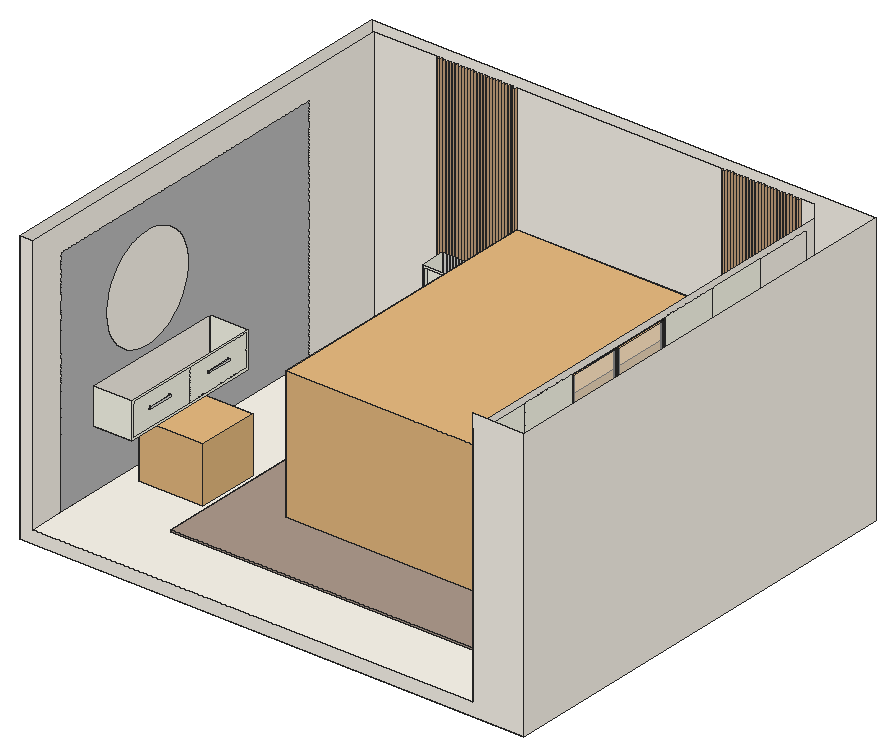
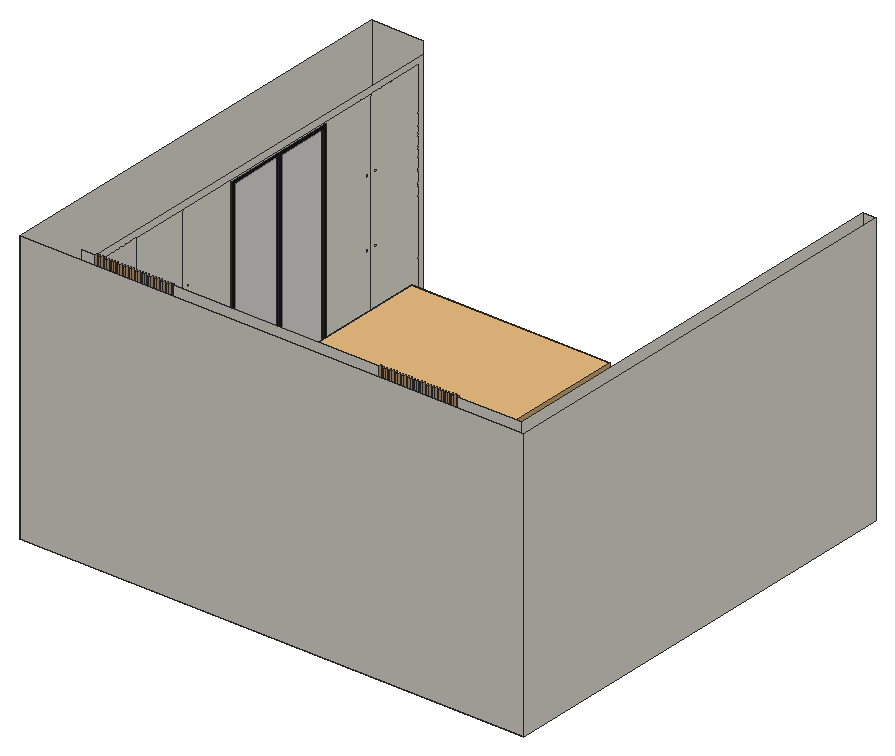
# SketchUp Ruby script. Lengths in inches.
U = 1.inch
M = Sketchup.active_model
def pt(a) = Geom::Point3d.new(a.map { |v| v * U })
def face(e, loops, mat)
  f = e.add_face(loops[0].map { |a| pt(a) })
  loops[1..].each { |l| e.add_face(l.map { |a| pt(a) }).erase! }
  f.material = f.back_material = mat if mat
  f
end
# faces: each face lists its corners as indices into pts; further lists are holes
def faces(e, pts, list, mat = nil) = list.each { |f| face(e, (f[0].is_a?(Array) ? f : [f]).map { |l| l.map { |i| pts[i] } }, mat) }
# xy, xz, yz: faces in a plane at the given z, y or x. An outline is a flat list of corners, or four numbers for a rectangle; further outlines are holes
def ring(l) = l.size == 4 ? [[l[0], l[1]], [l[2], l[1]], [l[2], l[3]], [l[0], l[3]]] : l.each_slice(2).to_a
def flat(e, list, mat, &to3) = list.each { |f| face(e, (f[0].is_a?(Array) ? f : [f]).map { |l| ring(l).map { |u, v| to3.(u, v) } }, mat) }
def xy(e, z, list, mat = nil) = flat(e, list, mat) { |x, y| [x, y, z] }
def xz(e, y, list, mat = nil) = flat(e, list, mat) { |x, z| [x, y, z] }
def yz(e, x, list, mat = nil) = flat(e, list, mat) { |y, z| [x, y, z] }
def lines(e, pts, list) = list.each { |a, b| e.add_line(pt(pts[a]), pt(pts[b])) }
# prism: a flat outline (further loops are holes) pulled along v
def prism(e, loops, v, mat = nil)
  f = face(e, loops, mat); d = Geom::Vector3d.new(v.map { |x| x * U })
  f.pushpull(f.normal.samedirection?(d) ? d.length : -d.length)
end
def box(e, o, s, mat = nil) = prism(e, [[o, [o[0] + s[0], o[1], o[2]], [o[0] + s[0], o[1] + s[1], o[2]], [o[0], o[1] + s[1], o[2]]]], [0, 0, s[2]], mat)
def at(x, y, z, deg = 0) = Geom::Transformation.translation(pt([x, y, z])) * Geom::Transformation.rotation(ORIGIN, Z_AXIS, deg.degrees)
def axes(o, x, y, z) = Geom::Transformation.new([*x, 0, *y, 0, *z, 0, *pt(o).to_a, 1])
def part(name) = M.definitions.add(name)
# library, detail: a bought-in or finely detailed component or shape, given as its bounding box
def library(name, o, s) = part(name).tap { |d| box(d.entities, o, s) }
def detail(e, o, s) = box(e.add_group.entities, o, s)
def put(e, d, t, mat = nil) = e.add_instance(d, t).tap { |i| i.material = mat if mat }
def group(e, t, mat = nil) = e.add_group.tap { |g| g.transformation = t; g.material = mat if mat }.entities
root = M.entities
M.materials.add("[0052_FloralWhite]").color = [255, 250, 240]
M.materials.add("[0053_Ivory]").color = [255, 255, 240]
M.materials.add("[Carpet Berber Multi]").color = [175, 156, 142]
M.materials.add("[Color M08]").color = [30, 30, 30]
M.materials.add("[Formica Laminate Light]").color = [219, 178, 137]
M.materials.add("[Suede Dark Gray]").color = [191, 191, 191]
M.materials.add("[Translucent Glass Blue]").color = [255, 255, 255]
M.materials["[Translucent Glass Blue]"].alpha = 0.5
c1 = library("Group",[-0.68,-0.68,0],[1.36,1.36,1.75])
c2 = library("Group\#6",[-3.9375,0,0],[90.55,70.87,32.69])
c3 = library("obj_04\#1",[-44.7,-42.95,7.39],[88.22,57.43,21.03])
c4 = library("Group\#14",[0,0,0],[78.74,62.99,7.09])
c5 = library("Group\#16",[0,0,0.9],[18.39,31.5,7.2])
c6 = library("Group\#17",[0,0,2],[18.39,30.67,6.07])
xy(root,0,[[0,0,234,204]],"[0052_FloralWhite]")
xy(root,6,[[63.36,197,64.8,198],[66.24,197,67.68,198],[69.12,197,70.56,198],[72,197,168,198],[169.44,197,170.88,198],
  [172.32,197,173.76,198],[175.2,197,176.64,198]])
xy(root,6,[[6,0,210,0,210,198,204,198,204,197,202.56,197,202.56,198,201.12,198,201.12,197,199.68,197,199.68,198,198.24,198,198.24,197,196.8,197,196.8,198,195.36,198,195.36,197,193.92,197,193.92,198,192.48,198,192.48,197,191.04,197,191.04,198,189.6,198,189.6,197,190.83,197,190.83,29.85,46.17,29.85,46.17,197,47.52,197,47.52,198,46.08,198,46.08,197,44.64,197,44.64,198,43.2,198,43.2,197,41.76,197,41.76,198,40.32,198,40.32,197,38.88,197,38.88,198,37.44,198,37.44,197,36,197,36,198,6,198]],"[0052_FloralWhite]")
xy(root,6,[[48.96,197,50.4,198],[51.84,197,53.28,198],[54.72,197,56.16,198],[57.6,197,59.04,198],[60.48,197,61.92,198],
  [178.08,197,179.52,198],[180.96,197,182.4,198],[183.84,197,185.28,198],[186.72,197,188.16,198]],"[0053_Ivory]")
xy(root,7,[[46.17,29.85,190.83,197]],"[Carpet Berber Multi]")
xy(root,9,[[209,57.57,210,84.86],[209,84.86,210,112.14]],"[Color M08]")
xy(root,10.5,[[209,59.07,210,83.36],[209,84.86,210,110.64]],"[Color M08]")
xy(root,28.16,[[38.88,185,38.88,197,69.12,197,69.12,185,68.12,185,68.12,186,39.88,186,39.88,185],[170.88,185,170.88,197,201.12,197,201.12,185,200.12,185,200.12,186,171.88,186,171.88,185]],"[0053_Ivory]")
xy(root,33.76,[[6,35.11,24,102.42]],"[0053_Ivory]")
xy(root,43.12,[[24.64,44.6,24.875,56.5],[24.64,78.6,24.875,90.5]])
xz(root,0,[[0,0,234,0,234,126,210,126,210,6,6,6,6,126,0,126]],"[0052_FloralWhite]")
xz(root,29.85,[[46.17,6,190.83,7]],"[Carpet Berber Multi]")
xz(root,35.11,[[6,33.76,24,50.39]],"[0053_Ivory]")
xz(root,44.6,[[24,42.79,24.64,43.12,24.875,43.12,24.875,43.79,24.64,43.79,24,44.13]])
xz(root,45.06,[[24,42.79,24,44.13,24.64,43.79,24.64,43.12]])
xz(root,56.04,[[24,42.79,24.64,43.12,24.64,43.79,24,44.13]])
xz(root,56.5,[[24,42.79,24,44.13,24.64,43.79,24.875,43.79,24.875,43.12,24.64,43.12]])
xz(root,57.57,[[209,9,210,117]],"[Color M08]")
xz(root,59.07,[[209,10.5,210,115.5]],"[Color M08]")
xz(root,78.6,[[24,42.79,24.64,43.12,24.875,43.12,24.875,43.79,24.64,43.79,24,44.13]])
xz(root,79.06,[[24,42.79,24,44.13,24.64,43.79,24.64,43.12]])
xz(root,83.36,[[209,10.5,210,115.5]],"[Color M08]")
xz(root,84.86,[[209,10.5,210,115.5]],"[Color M08]")
xz(root,90.04,[[24,42.79,24.64,43.12,24.64,43.79,24,44.13]])
xz(root,90.5,[[24,42.79,24,44.13,24.64,43.79,24.875,43.79,24.875,43.12,24.64,43.12]])
xz(root,102.42,[[6,33.76,24,50.39]],"[0053_Ivory]")
xz(root,110.64,[[209,10.5,210,115.5]],"[Color M08]")
xz(root,112.14,[[209,9,210,117]],"[Color M08]")
xz(root,185,[[38.88,28.16,39.88,28.16,39.88,45.24,68.12,45.24,68.12,28.16,69.12,28.16,69.12,46.24,38.88,46.24],[170.88,28.16,171.88,28.16,171.88,45.24,200.12,45.24,200.12,28.16,201.12,28.16,201.12,46.24,170.88,46.24]],"[0053_Ivory]")
xz(root,186,[[39.88,28.16,68.12,45.24],[171.88,28.16,200.12,45.24]],"[0053_Ivory]")
xz(root,197,[[72,6,168,7],[38.88,28.16,40.32,46.24],[40.32,28.16,41.76,46.24],[41.76,28.16,43.2,46.24],[43.2,28.16,44.64,46.24],
  [44.64,28.16,46.08,46.24],[46.08,28.16,47.52,46.24],[47.52,28.16,48.96,46.24],[48.96,28.16,50.4,46.24],[50.4,28.16,51.84,46.24],
  [51.84,28.16,53.28,46.24],[53.28,28.16,54.72,46.24],[54.72,28.16,56.16,46.24],[56.16,28.16,57.6,46.24],[57.6,28.16,59.04,46.24],
  [59.04,28.16,60.48,46.24],[60.48,28.16,61.92,46.24],[61.92,28.16,63.36,46.24],[63.36,28.16,64.8,46.24],[64.8,28.16,66.24,46.24],
  [66.24,28.16,67.68,46.24],[67.68,28.16,69.12,46.24],[170.88,28.16,172.32,46.24],[172.32,28.16,173.76,46.24],[173.76,28.16,175.2,46.24],
  [175.2,28.16,176.64,46.24],[176.64,28.16,178.08,46.24],[178.08,28.16,179.52,46.24],[179.52,28.16,180.96,46.24],[180.96,28.16,182.4,46.24],
  [182.4,28.16,183.84,46.24],[183.84,28.16,185.28,46.24],[185.28,28.16,186.72,46.24],[186.72,28.16,188.16,46.24],[188.16,28.16,189.6,46.24],
  [189.6,28.16,191.04,46.24],[191.04,28.16,192.48,46.24],[192.48,28.16,193.92,46.24],[193.92,28.16,195.36,46.24],[195.36,28.16,196.8,46.24],
  [196.8,28.16,198.24,46.24],[198.24,28.16,199.68,46.24],[199.68,28.16,201.12,46.24]])
xz(root,197,[[46.17,6,47.52,7],[48.96,6,50.4,7],[51.84,6,53.28,7],[54.72,6,56.16,7],[57.6,6,59.04,7],
  [60.48,6,61.92,7],[63.36,6,64.8,7],[66.24,6,67.68,7],[69.12,6,70.56,7],[169.44,6,170.88,7],
  [172.32,6,173.76,7],[175.2,6,176.64,7],[178.08,6,179.52,7],[180.96,6,182.4,7],[183.84,6,185.28,7],
  [186.72,6,188.16,7],[189.6,6,190.83,7]],"[Carpet Berber Multi]")
xz(root,197,[[36,6,37.44,126],[38.88,6,40.32,28.16],[41.76,6,43.2,28.16],[44.64,6,46.08,28.16],[47.52,6,48.96,7],
  [50.4,6,51.84,7],[53.28,6,54.72,7],[56.16,6,57.6,7],[59.04,6,60.48,7],[61.92,6,63.36,7],
  [64.8,6,66.24,7],[67.68,6,69.12,7],[70.56,6,72,7],[168,6,169.44,7],[170.88,6,172.32,7],
  [173.76,6,175.2,7],[176.64,6,178.08,7],[179.52,6,180.96,7],[182.4,6,183.84,7],[185.28,6,186.72,7],
  [188.16,6,189.6,7],[191.04,6,192.48,28.16],[193.92,6,195.36,28.16],[196.8,6,198.24,28.16],[199.68,6,201.12,28.16],
  [202.56,6,204,126],[47.52,7,48.96,28.16],[50.4,7,51.84,28.16],[53.28,7,54.72,28.16],[56.16,7,57.6,28.16],
  [59.04,7,60.48,28.16],[61.92,7,63.36,28.16],[64.8,7,66.24,28.16],[67.68,7,69.12,28.16],[70.56,7,72,126],
  [168,7,169.44,126],[170.88,7,172.32,28.16],[173.76,7,175.2,28.16],[176.64,7,178.08,28.16],[179.52,7,180.96,28.16],
  [182.4,7,183.84,28.16],[185.28,7,186.72,28.16],[188.16,7,189.6,28.16]],"[Formica Laminate Light]")
xz(root,198,[[6,6,36,126],[72,6,168,126],[204,6,210,126]],"[0052_FloralWhite]")
xz(root,198,[[37.44,6,38.88,126],[40.32,6,41.76,126],[43.2,6,44.64,126],[46.08,6,47.52,126],[48.96,6,50.4,126],
  [51.84,6,53.28,126],[54.72,6,56.16,126],[57.6,6,59.04,126],[60.48,6,61.92,126],[63.36,6,64.8,126],
  [66.24,6,67.68,126],[69.12,6,70.56,126],[169.44,6,170.88,126],[172.32,6,173.76,126],[175.2,6,176.64,126],
  [178.08,6,179.52,126],[180.96,6,182.4,126],[183.84,6,185.28,126],[186.72,6,188.16,126],[189.6,6,191.04,126],
  [192.48,6,193.92,126],[195.36,6,196.8,126],[198.24,6,199.68,126],[201.12,6,202.56,126]],"[Formica Laminate Light]")
xz(root,204,[[0,0,234,126]],"[0052_FloralWhite]")
yz(root,0,[[0,0,204,126]],"[0052_FloralWhite]")
yz(root,6,[[0,6,16.54,6,16.54,113.79,160.21,113.79,160.21,6,198,6,198,126,0,126]],"[0052_FloralWhite]")
yz(root,6,[[[16.54,6,160.21,113.79],[66.54,53.33,65.04,53.375,63.54,53.52,62.05,53.75,60.58,54.08,59.13,54.5,57.71,55.01,56.33,55.61,54.98,56.29,53.68,57.0625,52.4375,57.91,51.25,58.83,50.12,59.83,49.05,60.9,48.05,62.03,47.13,63.22,46.28,64.47,45.51,65.76,44.83,67.11,44.23,68.49,43.72,69.91,43.3,71.36,42.97,72.83,42.73,74.32,42.59,75.82,42.54,77.33,42.59,78.83,42.73,80.33,42.97,81.82,43.3,83.29,43.72,84.74,44.23,86.16,44.83,87.54,45.51,88.89,46.28,90.1875,47.13,91.43,48.05,92.625,49.05,93.75,50.12,94.82,51.25,95.82,52.4375,96.74,53.68,97.59,54.98,98.36,56.33,99.04,57.71,99.64,59.13,100.15,60.58,100.57,62.05,100.9,63.54,101.14,65.04,101.28,66.54,101.33,68.05,101.28,69.55,101.14,71.04,100.9,72.51,100.57,73.96,100.15,75.38,99.64,76.76,99.04,78.11,98.36,79.4,97.59,80.65,96.74,81.84,95.82,82.97,94.82,84.04,93.75,85.04,92.625,85.96,91.43,86.81,90.1875,87.58,88.89,88.26,87.54,88.86,86.16,89.37,84.74,89.79,83.29,90.12,81.82,90.36,80.33,90.5,78.83,90.54,77.33,90.5,75.82,90.36,74.32,90.12,72.83,89.79,71.36,89.37,69.91,88.86,68.49,88.26,67.11,87.58,65.76,86.81,64.47,85.96,63.22,85.04,62.03,84.04,60.9,82.97,59.83,81.84,58.83,80.65,57.91,79.4,57.0625,78.11,56.29,76.76,55.61,75.38,55.01,73.96,54.5,72.51,54.08,71.04,53.75,69.55,53.52,68.05,53.375],[35.11,33.76,102.42,50.39]]],"[Suede Dark Gray]")
yz(root,24,[[44.6,42.79,45.06,44.13],[56.04,42.79,56.5,44.13],[78.6,42.79,79.06,44.13],[90.04,42.79,90.5,44.13]])
yz(root,24,[[[35.11,33.76,102.42,50.39],[36.16,34.82,101.37,49.33]],[[36.16,34.82,68.77,49.33],[56.04,42.79,56.5,44.13],[44.6,42.79,45.06,44.13]],[[68.77,34.82,101.37,49.33],[78.6,42.79,79.06,44.13],[90.04,42.79,90.5,44.13]]],"[0053_Ivory]")
yz(root,24.64,[[45.06,43.12,56.04,43.79],[79.06,43.12,90.04,43.79]])
yz(root,24.875,[[44.6,43.12,56.5,43.79],[78.6,43.12,90.5,43.79]])
yz(root,36,[[197,6,198,126]],"[Formica Laminate Light]")
yz(root,37.44,[[197,6,198,126]],"[Formica Laminate Light]")
yz(root,38.88,[[185,28.16,197,46.24]],"[0053_Ivory]")
yz(root,38.88,[[197,6,198,126]],"[Formica Laminate Light]")
yz(root,39.88,[[185,28.16,186,45.24]],"[0053_Ivory]")
yz(root,40.32,[[197,6,198,126]],"[Formica Laminate Light]")
yz(root,41.76,[[197,6,198,126]],"[Formica Laminate Light]")
yz(root,43.2,[[197,6,198,126]],"[Formica Laminate Light]")
yz(root,44.64,[[197,6,198,126]],"[Formica Laminate Light]")
yz(root,46.08,[[197,6,198,126]],"[Formica Laminate Light]")
yz(root,46.17,[[29.85,6,197,7]],"[Carpet Berber Multi]")
yz(root,47.52,[[197,6,198,126]],"[Formica Laminate Light]")
yz(root,48.96,[[197,6,198,126]],"[Formica Laminate Light]")
yz(root,50.4,[[197,6,198,126]],"[Formica Laminate Light]")
yz(root,51.84,[[197,6,198,126]],"[Formica Laminate Light]")
yz(root,53.28,[[197,6,198,126]],"[Formica Laminate Light]")
yz(root,54.72,[[197,6,198,126]],"[Formica Laminate Light]")
yz(root,56.16,[[197,6,198,126]],"[Formica Laminate Light]")
yz(root,57.6,[[197,6,198,126]],"[Formica Laminate Light]")
yz(root,59.04,[[197,6,198,126]],"[Formica Laminate Light]")
yz(root,60.48,[[197,6,198,126]],"[Formica Laminate Light]")
yz(root,61.92,[[197,6,198,126]],"[Formica Laminate Light]")
yz(root,63.36,[[197,6,198,126]],"[Formica Laminate Light]")
yz(root,64.8,[[197,6,198,126]],"[Formica Laminate Light]")
yz(root,66.24,[[197,6,198,126]],"[Formica Laminate Light]")
yz(root,67.68,[[197,6,198,126]],"[Formica Laminate Light]")
yz(root,68.12,[[185,28.16,186,45.24]],"[0053_Ivory]")
yz(root,69.12,[[185,28.16,197,46.24]],"[0053_Ivory]")
yz(root,69.12,[[197,6,198,126]],"[Formica Laminate Light]")
yz(root,70.56,[[197,6,198,126]],"[Formica Laminate Light]")
yz(root,72,[[197,6,198,126]],"[Formica Laminate Light]")
yz(root,168,[[197,6,198,126]],"[Formica Laminate Light]")
yz(root,169.44,[[197,6,198,126]],"[Formica Laminate Light]")
yz(root,170.88,[[185,28.16,197,46.24]],"[0053_Ivory]")
yz(root,170.88,[[197,6,198,126]],"[Formica Laminate Light]")
yz(root,171.88,[[185,28.16,186,45.24]],"[0053_Ivory]")
yz(root,172.32,[[197,6,198,126]],"[Formica Laminate Light]")
yz(root,173.76,[[197,6,198,126]],"[Formica Laminate Light]")
yz(root,175.2,[[197,6,198,126]],"[Formica Laminate Light]")
yz(root,176.64,[[197,6,198,126]],"[Formica Laminate Light]")
yz(root,178.08,[[197,6,198,126]],"[Formica Laminate Light]")
yz(root,179.52,[[197,6,198,126]],"[Formica Laminate Light]")
yz(root,180.96,[[197,6,198,126]],"[Formica Laminate Light]")
yz(root,182.4,[[197,6,198,126]],"[Formica Laminate Light]")
yz(root,183.84,[[197,6,198,126]],"[Formica Laminate Light]")
yz(root,185.28,[[197,6,198,126]],"[Formica Laminate Light]")
yz(root,186.72,[[197,6,198,126]],"[Formica Laminate Light]")
yz(root,188.16,[[197,6,198,126]],"[Formica Laminate Light]")
yz(root,189.6,[[197,6,198,126]],"[Formica Laminate Light]")
yz(root,190.83,[[29.85,6,197,7]],"[Carpet Berber Multi]")
yz(root,191.04,[[197,6,198,126]],"[Formica Laminate Light]")
yz(root,192.48,[[197,6,198,126]],"[Formica Laminate Light]")
yz(root,193.92,[[197,6,198,126]],"[Formica Laminate Light]")
yz(root,195.36,[[197,6,198,126]],"[Formica Laminate Light]")
yz(root,196.8,[[197,6,198,126]],"[Formica Laminate Light]")
yz(root,198.24,[[197,6,198,126]],"[Formica Laminate Light]")
yz(root,199.68,[[197,6,198,126]],"[Formica Laminate Light]")
yz(root,200.12,[[185,28.16,186,45.24]],"[0053_Ivory]")
yz(root,201.12,[[185,28.16,197,46.24]],"[0053_Ivory]")
yz(root,201.12,[[197,6,198,126]],"[Formica Laminate Light]")
yz(root,202.56,[[197,6,198,126]],"[Formica Laminate Light]")
yz(root,204,[[197,6,198,126]],"[Formica Laminate Light]")
yz(root,209,[[[57.57,9,84.86,117],[59.07,10.5,83.36,115.5]],[84.86,9,84.86,10.5,110.64,10.5,110.64,115.5,84.86,115.5,84.86,117,112.14,117,112.14,9]],"[Color M08]")
yz(root,210,[[[0,6,198,120],[3,9,194,117]],[166.71,9,194,117]],"[0052_FloralWhite]")
yz(root,210,[[[3,9,30.29,117],[27.04,83.63,28.39,84.89],[27.04,52.34,28.39,53.6]],[[30.29,9,57.57,117],[32.23,83.63,33.58,84.89],[32.23,52.34,33.58,53.6]],[[112.14,9,139.43,117],[135.92,83.63,137.26,84.89],[135.92,52.34,137.26,53.6]],[[139.43,9,166.71,117],[141.92,83.63,143.26,84.89],[141.92,52.34,143.26,53.6]]],"[0053_Ivory]")
yz(root,210,[[59.07,10.5,83.36,115.5],[84.86,10.5,110.64,115.5]],"[Translucent Glass Blue]")
yz(root,234,[[0,0,204,126]],"[0052_FloralWhite]")
p = [[24.64,44.6,43.12],[24,44.6,42.79],[24,45.06,42.79],[24.64,45.06,43.12],[24.64,56.04,43.12],[24,56.04,42.79],
  [24,56.5,42.79],[24.64,56.5,43.12],[24.64,78.6,43.12],[24,78.6,42.79],[24,79.06,42.79],[24.64,79.06,43.12],
  [24.64,90.04,43.12],[24,90.04,42.79],[24,90.5,42.79],[24.64,90.5,43.12]]
faces(root,p,[[0,1,2,3],[4,5,6,7],[8,9,10,11],[12,13,14,15]])
put(root,c1,axes([28.48,66.46,6],[21.87405,0,0],[0,21.3,0],[0,0,14.72243]))
put(root,c2,axes([73.03,191.17,7.04],[0,-1.4803,0],[1.3,0,0],[0,0,1.8582]))
g1 = group(root,at(78.14,185.34,7.04))
prism(g1,[[[81.89,0,0],[81.89,-116.56,0],[0,-116.56,0],[0,0,0]],[[0.92,-115.51,0],[80.97,-115.51,0],[80.97,-1.05,0],[0.92,-1.05,0]]],[0,0,18.29])
put(root,c3,axes([120.1875,125.49,1.74],[-1.23416,0,0],[0,1.1845,0],[0,0,1.8582]))
put(root,c4,axes([78.14,185.34,25.51],[0,-1.4803,0],[1.3,0,0],[0,0,1.8582]))
put(root,c5,axes([121.28,187.14,40.83],[0,-1.39965,-0.60497],[1.14266,0,0],[0,-0.48194,1.75696]))
put(root,c6,axes([81.47,186.97,39.57],[0,-1.42986,-0.48094],[1.17,0,0],[0,-0.38313,1.79488]))
